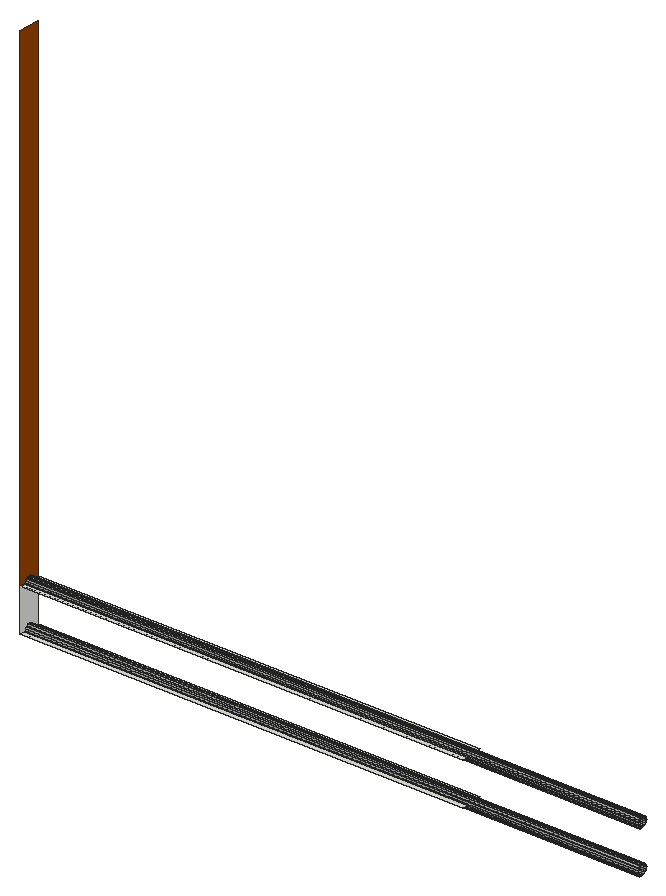
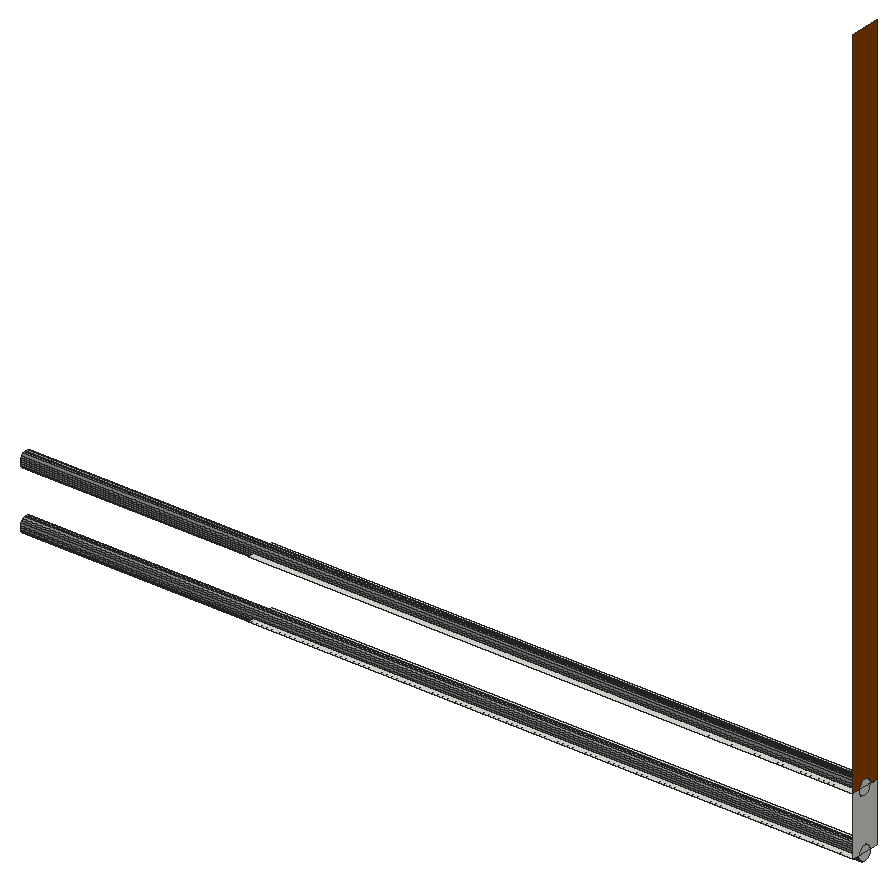
# SketchUp Ruby script. Lengths in inches.
U = 1.inch
M = Sketchup.active_model
def pt(a) = Geom::Point3d.new(a.map { |v| v * U })
def face(e, loops, mat)
  f = e.add_face(loops[0].map { |a| pt(a) })
  loops[1..].each { |l| e.add_face(l.map { |a| pt(a) }).erase! }
  f.material = f.back_material = mat if mat
  f
end
# faces: each face lists its corners as indices into pts; further lists are holes
def faces(e, pts, list, mat = nil) = list.each { |f| face(e, (f[0].is_a?(Array) ? f : [f]).map { |l| l.map { |i| pts[i] } }, mat) }
# xy, xz, yz: faces in a plane at the given z, y or x. An outline is a flat list of corners, or four numbers for a rectangle; further outlines are holes
def ring(l) = l.size == 4 ? [[l[0], l[1]], [l[2], l[1]], [l[2], l[3]], [l[0], l[3]]] : l.each_slice(2).to_a
def flat(e, list, mat, &to3) = list.each { |f| face(e, (f[0].is_a?(Array) ? f : [f]).map { |l| ring(l).map { |u, v| to3.(u, v) } }, mat) }
def xy(e, z, list, mat = nil) = flat(e, list, mat) { |x, y| [x, y, z] }
def xz(e, y, list, mat = nil) = flat(e, list, mat) { |x, z| [x, y, z] }
def yz(e, x, list, mat = nil) = flat(e, list, mat) { |y, z| [x, y, z] }
def lines(e, pts, list) = list.each { |a, b| e.add_line(pt(pts[a]), pt(pts[b])) }
# prism: a flat outline (further loops are holes) pulled along v
def prism(e, loops, v, mat = nil)
  f = face(e, loops, mat); d = Geom::Vector3d.new(v.map { |x| x * U })
  f.pushpull(f.normal.samedirection?(d) ? d.length : -d.length)
end
def box(e, o, s, mat = nil) = prism(e, [[o, [o[0] + s[0], o[1], o[2]], [o[0] + s[0], o[1] + s[1], o[2]], [o[0], o[1] + s[1], o[2]]]], [0, 0, s[2]], mat)
def at(x, y, z, deg = 0) = Geom::Transformation.translation(pt([x, y, z])) * Geom::Transformation.rotation(ORIGIN, Z_AXIS, deg.degrees)
def axes(o, x, y, z) = Geom::Transformation.new([*x, 0, *y, 0, *z, 0, *pt(o).to_a, 1])
def part(name) = M.definitions.add(name)
# library, detail: a bought-in or finely detailed component or shape, given as its bounding box
def library(name, o, s) = part(name).tap { |d| box(d.entities, o, s) }
def detail(e, o, s) = box(e.add_group.entities, o, s)
def put(e, d, t, mat = nil) = e.add_instance(d, t).tap { |i| i.material = mat if mat }
def group(e, t, mat = nil) = e.add_group.tap { |g| g.transformation = t; g.material = mat if mat }.entities
root = M.entities
M.materials.add("[0132_LightGray]").color = [169, 169, 169]
M.materials.add("[Wood Cherry Original]").color = [152, 68, 0]
xy(root,86.51,[[61.9375,82.25,103.25,84.25]])
xy(root,90.51,[[61.9375,82.25,103.25,84.25]])
yz(root,61.9375,[[83.25,85.96,83.38,85.98,83.5,86.03,83.6,86.11,83.68,86.21,83.73,86.34,83.75,86.46,83.74,86.51,82.76,86.51,82.75,86.46,82.77,86.34,82.82,86.21,82.9,86.11,83,86.03,83.12,85.98],[82.25,86.51,82.76,86.51,82.77,86.59,82.82,86.71,82.9,86.82,83,86.9,83.12,86.95,83.25,86.96,83.38,86.95,83.5,86.9,83.6,86.82,83.68,86.71,83.73,86.59,83.74,86.51,84.25,86.51,84.25,90.51,83.74,90.51,83.75,90.46,83.73,90.34,83.68,90.21,83.6,90.11,83.5,90.03,83.38,89.98,83.25,89.96,83.12,89.98,83,90.03,82.9,90.11,82.82,90.21,82.77,90.34,82.75,90.46,82.76,90.51,82.25,90.51],[82.76,86.51,83.74,86.51,83.73,86.59,83.68,86.71,83.6,86.82,83.5,86.9,83.38,86.95,83.25,86.96,83.12,86.95,83,86.9,82.9,86.82,82.82,86.71,82.77,86.59],[83.25,89.96,83.38,89.98,83.5,90.03,83.6,90.11,83.68,90.21,83.73,90.34,83.75,90.46,83.74,90.51,82.76,90.51,82.75,90.46,82.77,90.34,82.82,90.21,82.9,90.11,83,90.03,83.12,89.98],[82.76,90.51,83.74,90.51,83.73,90.59,83.68,90.71,83.6,90.82,83.5,90.9,83.38,90.95,83.25,90.96,83.12,90.95,83,90.9,82.9,90.82,82.82,90.71,82.77,90.59]])
yz(root,61.9375,[[82.25,90.51,82.76,90.51,82.77,90.59,82.82,90.71,82.9,90.82,83,90.9,83.12,90.95,83.25,90.96,83.38,90.95,83.5,90.9,83.6,90.82,83.68,90.71,83.73,90.59,83.74,90.51,84.25,90.51,84.25,137.01,82.25,137.01]],"[Wood Cherry Original]")
p = [[119.25,83,86.03],[119.25,82.9,86.11],[61.9375,82.9,86.11],[61.9375,83,86.03],[119.25,83.12,85.98],[61.9375,83.12,85.98],
  [119.25,83.25,85.96],[61.9375,83.25,85.96],[119.25,83.38,85.98],[61.9375,83.38,85.98],[119.25,83.5,86.03],[61.9375,83.5,86.03],
  [119.25,83.6,86.11],[61.9375,83.6,86.11],[119.25,82.82,86.21],[61.9375,82.82,86.21],[119.25,83.68,86.21],[61.9375,83.68,86.21],
  [119.25,82.77,86.34],[61.9375,82.77,86.34],[119.25,83.73,86.34],[61.9375,83.73,86.34],[119.25,82.75,86.46],[61.9375,82.75,86.46],
  [119.25,83.75,86.46],[61.9375,83.75,86.46],[119.25,82.77,86.59],[61.9375,82.77,86.59],[61.9375,82.76,86.51],[119.25,83.73,86.59],
  [61.9375,83.74,86.51],[61.9375,83.73,86.59],[119.25,82.82,86.71],[61.9375,82.82,86.71],[119.25,83.68,86.71],[61.9375,83.68,86.71],
  [119.25,82.9,86.82],[61.9375,82.9,86.82],[119.25,83.6,86.82],[61.9375,83.6,86.82],[119.25,83,86.9],[61.9375,83,86.9],
  [119.25,83.5,86.9],[61.9375,83.5,86.9],[119.25,83.12,86.95],[61.9375,83.12,86.95],[119.25,83.25,86.96],[61.9375,83.25,86.96],
  [119.25,83.38,86.95],[61.9375,83.38,86.95],[119.25,83,90.03],[119.25,82.9,90.11],[61.9375,82.9,90.11],[61.9375,83,90.03],
  [119.25,83.12,89.98],[61.9375,83.12,89.98],[119.25,83.25,89.96],[61.9375,83.25,89.96],[119.25,83.38,89.98],[61.9375,83.38,89.98],
  [119.25,83.5,90.03],[61.9375,83.5,90.03],[119.25,83.6,90.11],[61.9375,83.6,90.11],[119.25,82.82,90.21],[61.9375,82.82,90.21],
  [119.25,83.68,90.21],[61.9375,83.68,90.21],[119.25,82.77,90.34],[61.9375,82.77,90.34],[119.25,83.73,90.34],[61.9375,83.73,90.34],
  [119.25,82.75,90.46],[61.9375,82.75,90.46],[119.25,83.75,90.46],[61.9375,83.75,90.46],[119.25,82.77,90.59],[61.9375,82.77,90.59],
  [61.9375,82.76,90.51],[119.25,83.73,90.59],[61.9375,83.74,90.51],[61.9375,83.73,90.59],[119.25,82.82,90.71],[61.9375,82.82,90.71],
  [119.25,83.68,90.71],[61.9375,83.68,90.71],[119.25,82.9,90.82],[61.9375,82.9,90.82],[119.25,83.6,90.82],[61.9375,83.6,90.82],
  [119.25,83,90.9],[61.9375,83,90.9],[119.25,83.5,90.9],[61.9375,83.5,90.9],[119.25,83.12,90.95],[61.9375,83.12,90.95],
  [119.25,83.25,90.96],[61.9375,83.25,90.96],[119.25,83.38,90.95],[61.9375,83.38,90.95]]
faces(root,p,[[0,1,2,3],[4,0,3,5],[6,4,5,7],[8,6,7,9],[10,8,9,11],[12,10,11,13],[1,14,15,2],[16,12,13,17],
  [14,18,19,15],[20,16,17,21],[18,22,23,19],[24,20,21,25],[22,26,27,28,23],[29,24,25,30,31],[26,32,33,27],[34,29,31,35],
  [32,36,37,33],[38,34,35,39],[36,40,41,37],[42,38,39,43],[40,44,45,41],[44,46,47,45],[46,48,49,47],[48,42,43,49],
  [50,51,52,53],[54,50,53,55],[56,54,55,57],[58,56,57,59],[60,58,59,61],[62,60,61,63],[51,64,65,52],[66,62,63,67],
  [64,68,69,65],[70,66,67,71],[68,72,73,69],[74,70,71,75],[72,76,77,78,73],[79,74,75,80,81],[76,82,83,77],[84,79,81,85],
  [82,86,87,83],[88,84,85,89],[86,90,91,87],[92,88,89,93],[90,94,95,91],[94,96,97,95],[98,92,93,99]],"[0132_LightGray]")
